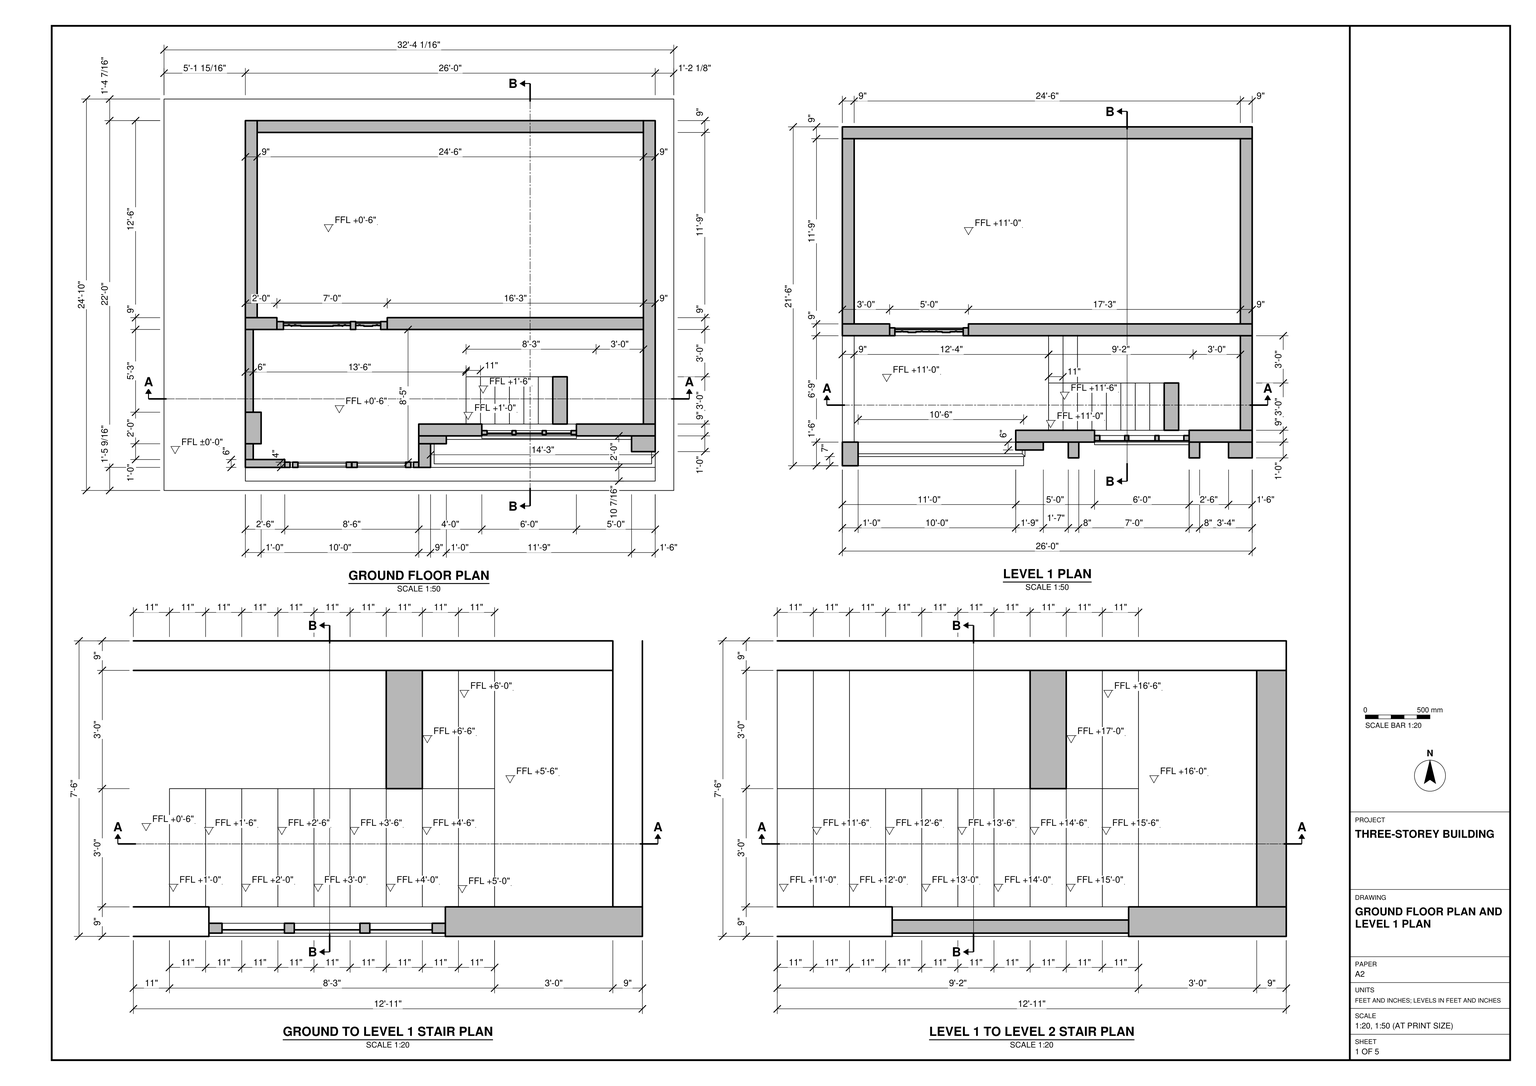
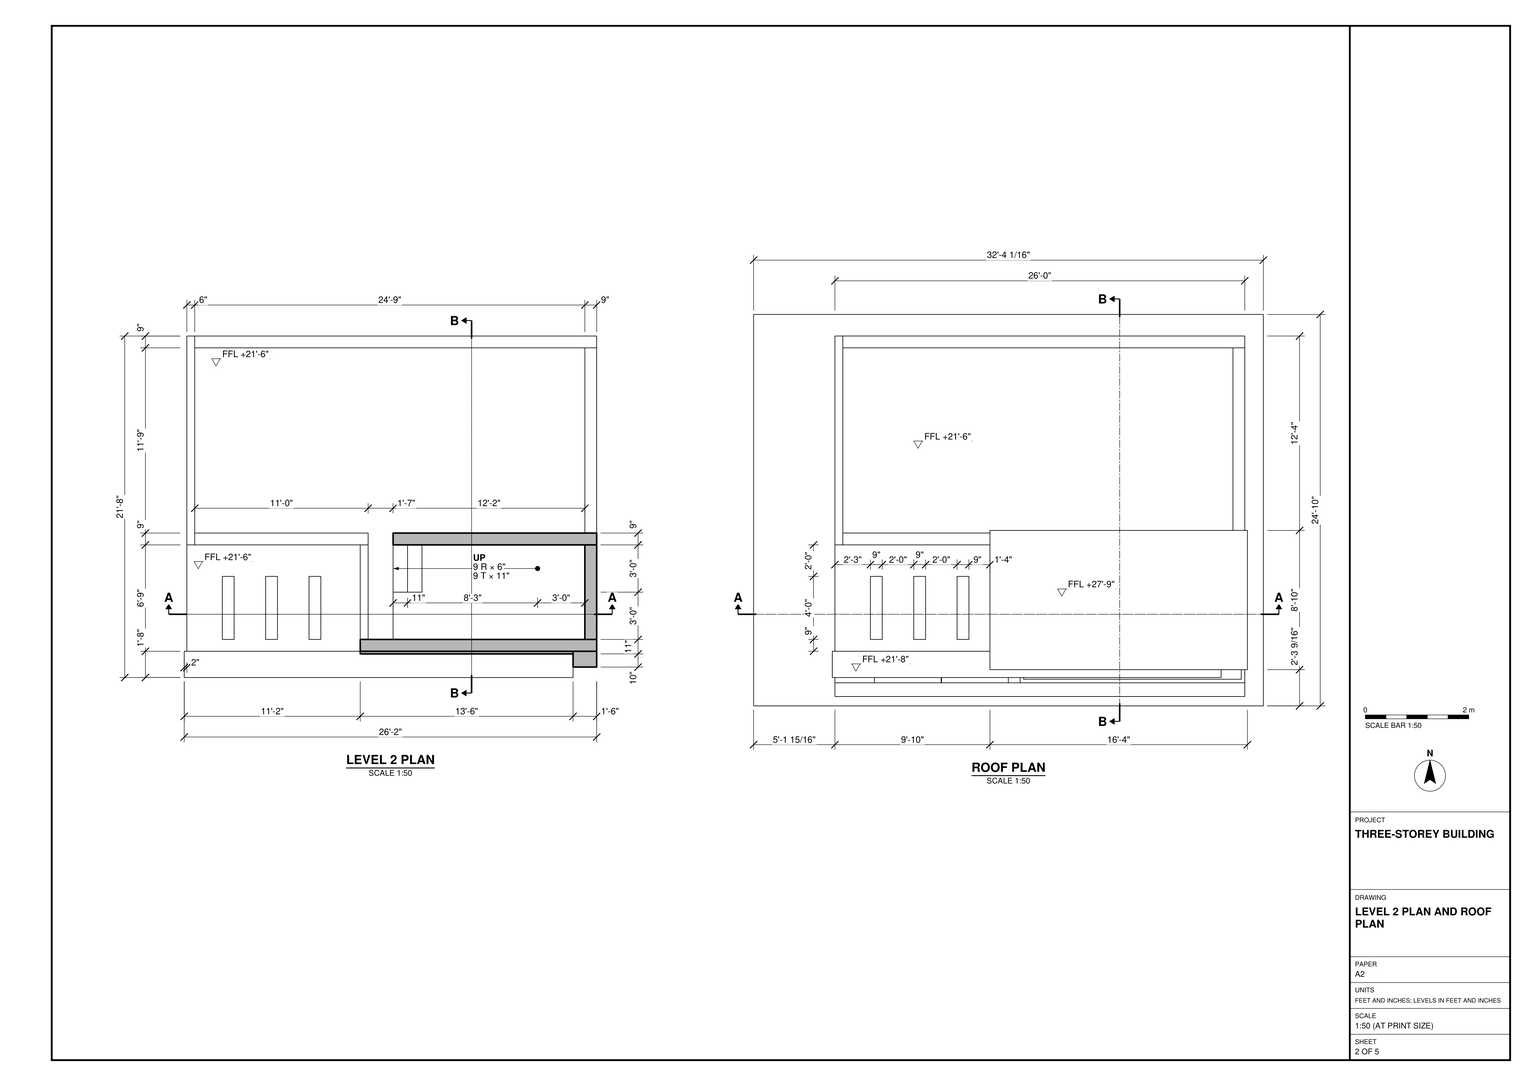
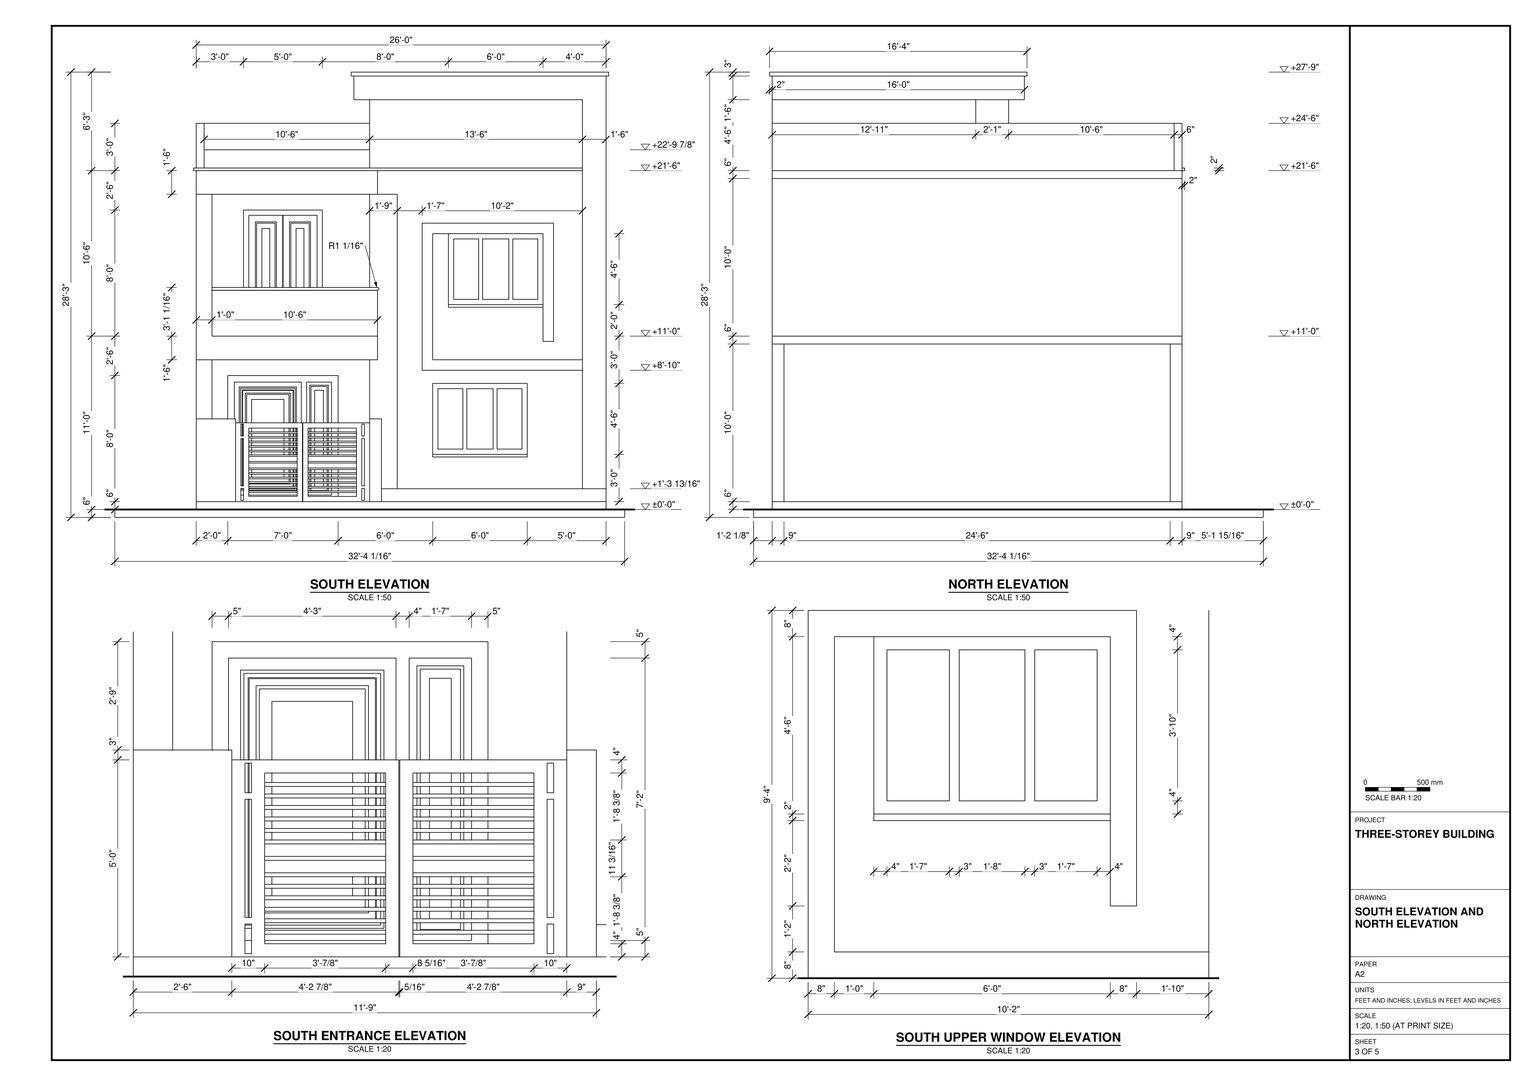
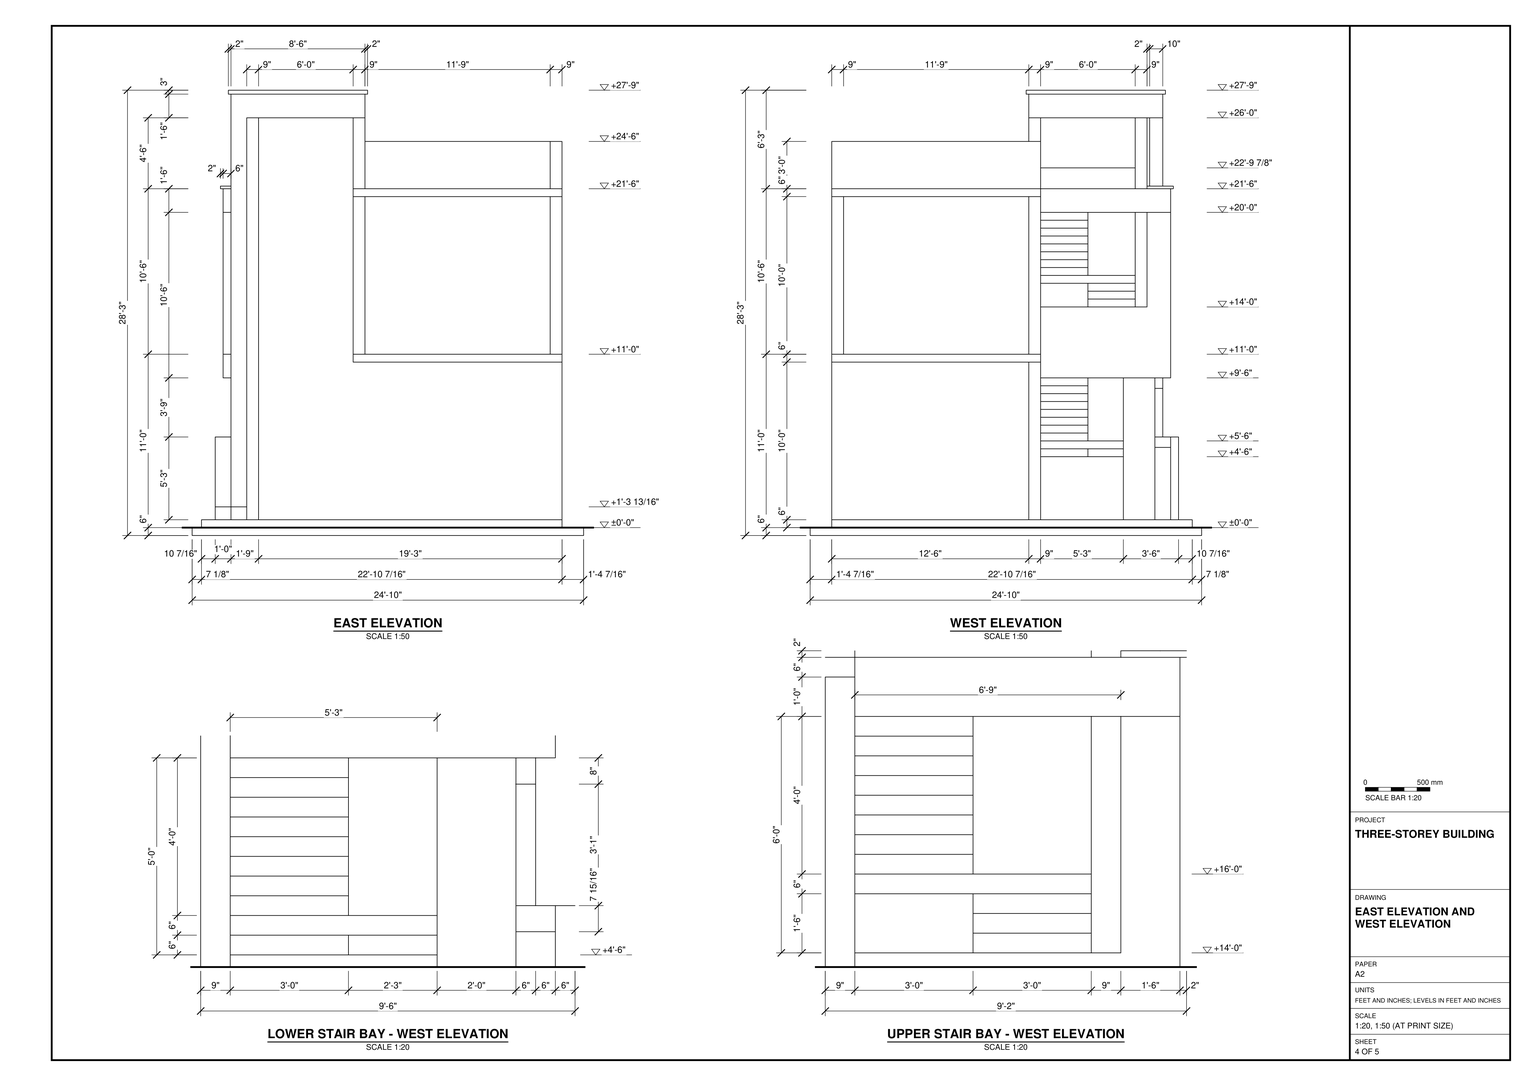
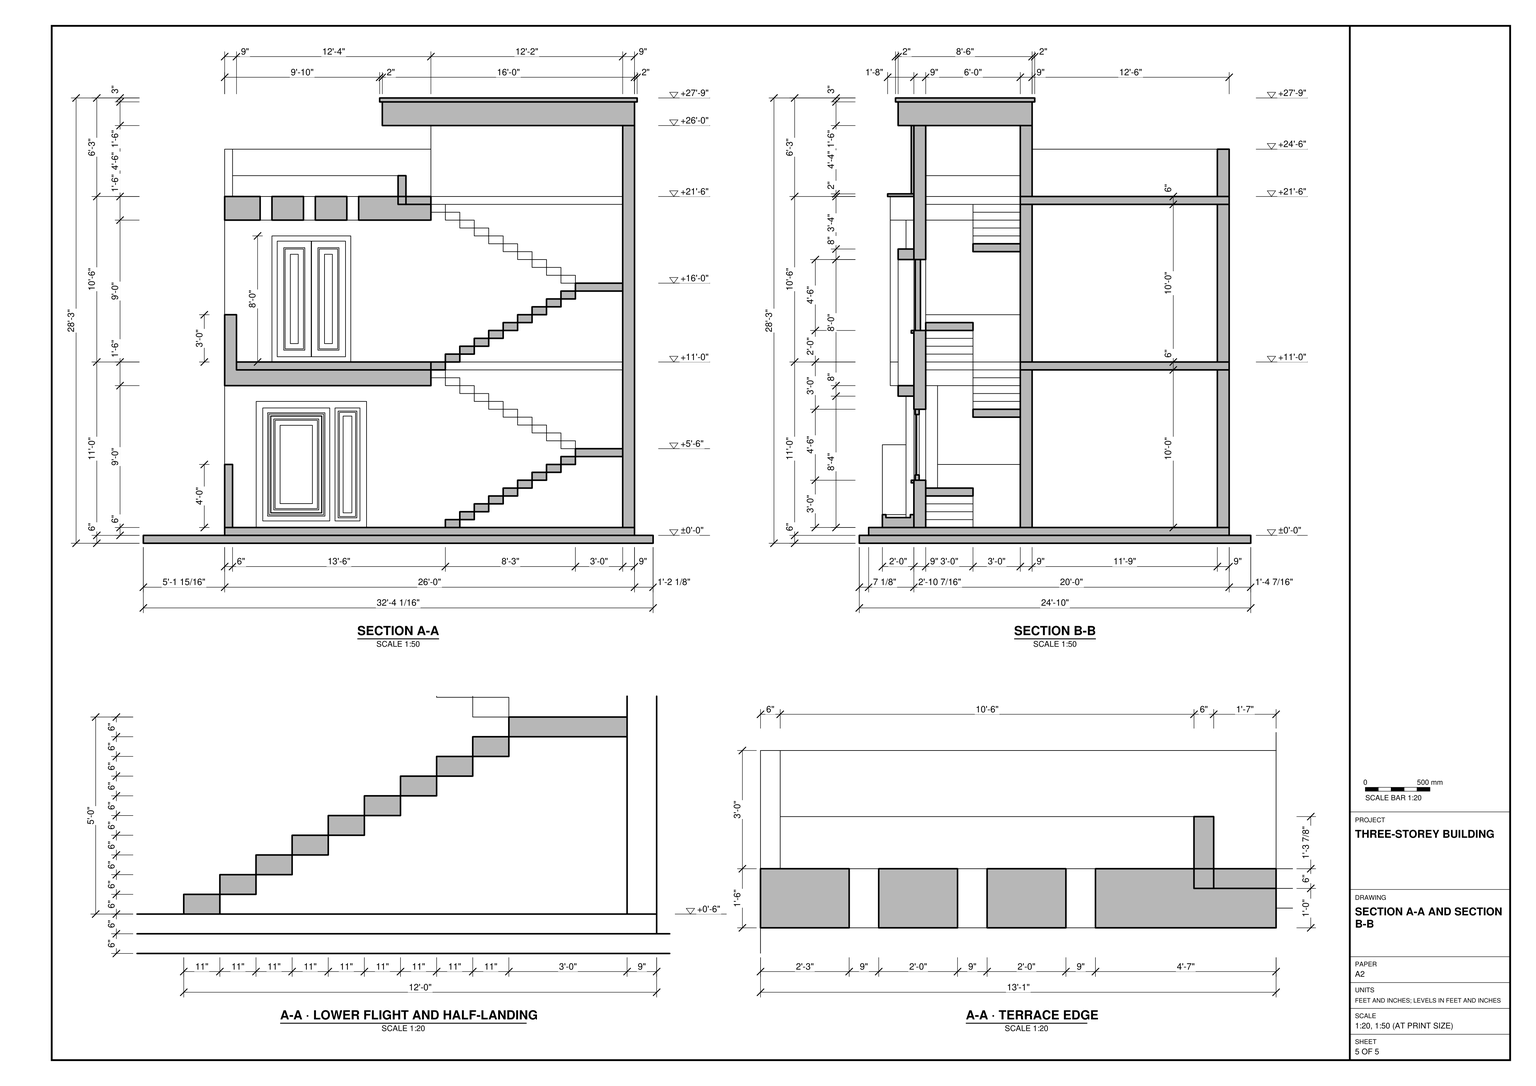
Build the three-storey building in SketchUp using task_files/diagram_01.pdf. Work in feet and inches. Including the base, the model must measure 32'-4 1/16" along X, 24'-10" along Y and 28'-3" along Z. Use ±0'-0" as the ground datum, with Level 1 at +11'-0" and Level 2 at +21'-6". Set the ground-floor finished surface at +0'-6" where marked.

Position the 26'-0" wide building on the base with the larger side setback to the west. On the ground floor and Level 1, form the full-width rear room and the front entrance and stair bays. Model the slabs and walls at their drawn thicknesses, distinguishing the 9" walls from the 6" walls. Follow the separate stair plans for the returning flights and landings so the stairs connect both floors to the roof terrace.

On the south elevation, place the slatted entrance gate in front of the recessed doorway and the balcony above it. Model the divided windows in the right-hand bay, including the projecting surround at the upper window. Finish the terrace with its parapets and the raised flat roof over the stair.

Keep walls, slabs, stairs, roof elements and any furniture or joinery pieces in separate groups or components; use components for repeated parts. Any decor or loose items shown may be suitable library components. Save one SketchUp model as output_files/three_storey_building_with_its_stair_and_roof_terrace.skp.

# SketchUp Ruby script. Lengths in inches.
U = 1.inch
M = Sketchup.active_model
def pt(a) = Geom::Point3d.new(a.map { |v| v * U })
def face(e, loops, mat)
  f = e.add_face(loops[0].map { |a| pt(a) })
  loops[1..].each { |l| e.add_face(l.map { |a| pt(a) }).erase! }
  f.material = f.back_material = mat if mat
  f
end
# faces: each face lists its corners as indices into pts; further lists are holes
def faces(e, pts, list, mat = nil) = list.each { |f| face(e, (f[0].is_a?(Array) ? f : [f]).map { |l| l.map { |i| pts[i] } }, mat) }
# xy, xz, yz: faces in a plane at the given z, y or x. An outline is a flat list of corners, or four numbers for a rectangle; further outlines are holes
def ring(l) = l.size == 4 ? [[l[0], l[1]], [l[2], l[1]], [l[2], l[3]], [l[0], l[3]]] : l.each_slice(2).to_a
def flat(e, list, mat, &to3) = list.each { |f| face(e, (f[0].is_a?(Array) ? f : [f]).map { |l| ring(l).map { |u, v| to3.(u, v) } }, mat) }
def xy(e, z, list, mat = nil) = flat(e, list, mat) { |x, y| [x, y, z] }
def xz(e, y, list, mat = nil) = flat(e, list, mat) { |x, z| [x, y, z] }
def yz(e, x, list, mat = nil) = flat(e, list, mat) { |y, z| [x, y, z] }
def lines(e, pts, list) = list.each { |a, b| e.add_line(pt(pts[a]), pt(pts[b])) }
# prism: a flat outline (further loops are holes) pulled along v
def prism(e, loops, v, mat = nil)
  f = face(e, loops, mat); d = Geom::Vector3d.new(v.map { |x| x * U })
  f.pushpull(f.normal.samedirection?(d) ? d.length : -d.length)
end
def box(e, o, s, mat = nil) = prism(e, [[o, [o[0] + s[0], o[1], o[2]], [o[0] + s[0], o[1] + s[1], o[2]], [o[0], o[1] + s[1], o[2]]]], [0, 0, s[2]], mat)
def at(x, y, z, deg = 0) = Geom::Transformation.translation(pt([x, y, z])) * Geom::Transformation.rotation(ORIGIN, Z_AXIS, deg.degrees)
def axes(o, x, y, z) = Geom::Transformation.new([*x, 0, *y, 0, *z, 0, *pt(o).to_a, 1])
def part(name) = M.definitions.add(name)
# library, detail: a bought-in or finely detailed component or shape, given as its bounding box
def library(name, o, s) = part(name).tap { |d| box(d.entities, o, s) }
def detail(e, o, s) = box(e.add_group.entities, o, s)
def put(e, d, t, mat = nil) = e.add_instance(d, t).tap { |i| i.material = mat if mat }
def group(e, t, mat = nil) = e.add_group.tap { |g| g.transformation = t; g.material = mat if mat }.entities
root = M.entities
M.materials.add("[Color E01]").color = [255, 255, 204]
M.materials.add("[Color M00]").color = [255, 255, 255]
M.materials.add("[Color M06]").color = [86, 86, 86]
M.materials.add("[Color M07]").color = [58, 58, 58]
M.materials.add("[Color M08]").color = [30, 30, 30]
M.materials.add("[Concrete Block Retaining Gray]").color = [121, 121, 121]
M.materials.add("[Grass Dark Green]").color = [106, 157, 55]
M.materials.add("[Pavers Modular Brick]").color = [158, 100, 89]
M.materials.add("[Translucent Glass Blue]").color = [100, 149, 237]
M.materials["[Translucent Glass Blue]"].alpha = 0.5
M.materials.add("[Wood Veneer 01]").color = [86, 50, 26]
c1 = part("Group\#5")
box(c1.entities,[0,0,0],[36,72,6])
c2 = part("Group\#4")
box(c2.entities,[0,0,0],[11,36,6])
c3 = part("Group\#60")
box(c3.entities,[0,1,0],[36.85,2,1.2])
c4 = part("Group\#58")
box(c4.entities,[0,1,0],[36.85,2,1.2])
c5 = part("Group\#62")
box(c5.entities,[0,1,0],[36.85,2,1.2])
c6 = part("Group\#59")
box(c6.entities,[0,1,0],[36.85,2,1.2])
p = [[199.92,35.57,138],[193.92,35.57,138],[193.92,41.57,138],[73.92,31.63,174],[199.92,31.63,174],[199.92,35.57,174],
  [199.92,35.57,120],[193.92,35.57,120],[193.92,50.57,120],[199.92,50.57,120]]
lines(root,p,[[0,1],[1,2],[3,4],[4,5],[6,7],[7,8],[8,9],[0,6]])
g1 = group(root,at(72,33,0))
box(g1,[-72,-33,0],[388.0625,298,6])
g2 = group(root,at(229.92,41.57,12),"[Color M06]")
prism(g2,[[[-36,0,0],[144,0,0],[144,0,306],[-36,0,306]],[[12,0,90],[84,0,90],[84,0,36],[12,0,36]],[[24,0,150],[24,0,204],[96,0,204],[96,0,150]]],[0,9,0])
g3 = group(root,at(364.92,50.57,12),"[Color E01]")
prism(g3,[[[0,231,0],[0,0,0],[0,0,306],[0,72,306],[0,72,120],[0,231,120]]],[9,0,0])
g4 = group(root,at(109.92,122.57,12),"[Color E01]")
prism(g4,[[[255,9,120],[255,9,0],[60,9,0],[60,9,96],[-24,9,96],[-24,9,0],[-48,9,0],[-48,9,120]]],[0,-9,0])
g5 = group(root,at(218.92,50.57,12))
put(g5,c1,at(110,0,54))
g6 = group(g5,at(11,0,0))
put(g6,c2,at(66,0,36))
put(g6,c2,at(88,0,48))
put(g6,c2,at(0,0,0))
put(g6,c2,at(77,0,42))
put(g6,c2,at(11,0,6))
put(g6,c2,at(55,0,30))
put(g6,c2,at(22,0,12))
put(g6,c2,at(33,0,18))
put(g6,c2,at(44,0,24))
put(g5,c2,at(22,72,108,180))
put(g5,c2,at(55,72,90,180))
put(g5,c2,at(44,72,96,180))
put(g5,c2,at(99,72,66,180))
put(g5,c2,at(110,72,60,180))
put(g5,c2,at(77,72,78,180))
put(g5,c2,at(33,72,102,180))
put(g5,c2,at(88,72,72,180))
put(g5,c2,at(66,72,84,180))
put(g5,c2,at(11,72,114,180))
g7 = group(root,at(109.92,122.57,132),"[Color E01]")
prism(g7,[[[264,0,0],[109,0,0],[109,-72,0],[84,-72,0],[84,-81,0],[-39,-81,0],[-39,0,0],[-48,0,0],[-48,159,0],[264,159,0]]],[0,0,6])
put(root,c2,at(317.92,122.57,204,180))
put(root,c2,at(273.92,122.57,228,180))
put(root,c2,at(251.92,122.57,240,180))
put(root,c2,at(240.92,122.57,246,180))
put(root,c2,at(284.92,122.57,222,180))
put(root,c2,at(306.92,122.57,210,180))
put(root,c2,at(295.92,122.57,216,180))
put(root,c2,at(328.92,122.57,198,180))
put(root,c2,at(262.92,122.57,234,180))
put(root,c1,at(328.92,50.57,192))
put(root,c2,at(229.92,122.57,252,180))
put(root,c2,at(295.92,50.57,174))
put(root,c2,at(240.92,50.57,144))
put(root,c2,at(251.92,50.57,150))
put(root,c2,at(262.92,50.57,156))
put(root,c2,at(317.92,50.57,186))
put(root,c2,at(284.92,50.57,168))
put(root,c2,at(273.92,50.57,162))
put(root,c2,at(229.92,50.57,138))
put(root,c2,at(306.92,50.57,180))
put(root,c2,at(218.92,50.57,132))
g8 = group(root,at(109.92,122.57,138),"[Color E01]")
prism(g8,[[[-12,9,0],[-48,9,0],[-48,9,120],[264,9,120],[264,9,0],[48,9,0],[48,9,96],[-12,9,96]]],[0,-9,0])
g9 = group(root,at(109.92,272.57,138),"[Color E01]")
box(g9,[-48,0,0],[312,9,120])
g10 = group(root,at(364.92,131.57,138),"[Color E01]")
box(g10,[0,0,0],[9,141,120])
g11 = group(root,at(109.92,122.57,258),"[Color E01]")
prism(g11,[[[264,159,0],[264,0,0],[109,0,0],[109,-72,0],[84,-72,0],[84,0,0],[-48,0,0],[-48,159,0]]],[0,0,6])
g12 = group(root,at(241.92,41.57,48),"[Color M08]")
prism(g12,[[[0,4,54],[72,4,54],[72,4,0],[0,4,0]],[[26,4,4],[46,4,4],[46,4,50],[26,4,50]],[[23,4,4],[23,4,50],[4,4,50],[4,4,4]],[[49,4,50],[49,4,4],[68,4,4],[68,4,50]]],[0,-3,0])
g13 = group(root,at(290.92,43.57,52),"[Translucent Glass Blue]")
xz(g13,0,[[0,0,19,46]])
g14 = group(root,at(267.92,43.57,52),"[Translucent Glass Blue]")
xz(g14,0,[[0,0,20,46]])
g15 = group(root,at(245.92,43.57,52),"[Translucent Glass Blue]")
xz(g15,0,[[0,0,19,46]])
g16 = group(root,at(109.92,41.57,120),"[Color E01]")
xy(g16,0,[[-48,-18,-48,81,109,81,109,9,90,9,90,-18]])
xy(g16,12,[[-39,0,90,0,90,9,109,9,109,81,-39,81]])
xy(g16,18,[[-36,-18,90,0]])
xy(g16,54,[[-48,0,-39,81]])
xy(g16,126,[[-48,-18,-36,0]])
xz(g16,-18,[[-48,0,90,0,90,18,-36,18,-36,126,-48,126]])
xz(g16,0,[[-39,12,-39,54,-48,54,-48,126,-36,126,-36,18,90,18,90,12]])
xz(g16,9,[[90,0,109,12]])
xz(g16,81,[[-48,0,-48,54,-39,54,-39,12,109,12,109,0]])
yz(g16,-48,[[-18,0,-18,126,0,126,0,54,81,54,81,0]])
yz(g16,-39,[[0,12,81,54]])
yz(g16,-36,[[-18,18,0,126]])
yz(g16,90,[[-18,0,9,0,9,12,0,12,0,18,-18,18]])
yz(g16,109,[[9,0,81,12]])
g17 = group(root,at(85.92,122.57,12),"[Wood Veneer 01]")
prism(g17,[[[84,6,0],[0,6,0],[0,6,96],[84,6,96]],[[56,6,5],[56,6,91],[5,6,91],[5,6,5]],[[79,6,91],[60,6,91],[60,6,5],[79,6,5]]],[0,-6,0])
g18 = group(root,at(90.92,125.07,17),"[Wood Veneer 01]")
xy(g18,0,[[0,0.5,51,2.5]])
xy(g18,3.67,[[3.67,0.5,47.33,1]])
xy(g18,4.67,[[4.67,0.5,46.33,1]])
xy(g18,5.96,[[5.96,0,45.04,0.5]])
xy(g18,6.28,[[6.28,0,44.72,0.5]])
xy(g18,8.39,[[8.39,0.5,42.61,1]])
xy(g18,9.39,[[9.39,0.5,41.61,1]])
xy(g18,13.2,[[13.2,0,37.8,0.5]])
xy(g18,72.8,[[13.2,0,37.8,0.5]])
xy(g18,76.61,[[9.39,0.5,41.61,1]])
xy(g18,77.61,[[8.39,0.5,42.61,1]])
xy(g18,79.72,[[6.28,0,44.72,0.5]])
xy(g18,80.04,[[5.96,0,45.04,0.5]])
xy(g18,81.33,[[4.67,0.5,46.33,1]])
xy(g18,82.33,[[3.67,0.5,47.33,1]])
xy(g18,86,[[0,0.5,51,2.5]])
xz(g18,0,[[[5.96,5.96,45.04,80.04],[6.28,6.28,44.72,79.72]],[13.2,13.2,37.8,72.8]])
xz(g18,0.5,[[[0,0,51,86],[3.67,3.67,47.33,82.33]],[[4.67,4.67,46.33,81.33],[5.96,5.96,45.04,80.04]],[[6.28,6.28,44.72,79.72],[8.39,8.39,42.61,77.61]],[[9.39,9.39,41.61,76.61],[13.2,13.2,37.8,72.8]]])
xz(g18,1,[[[3.67,3.67,47.33,82.33],[4.67,4.67,46.33,81.33]],[[8.39,8.39,42.61,77.61],[9.39,9.39,41.61,76.61]]])
xz(g18,2.5,[[0,0,51,86]])
yz(g18,0,[[0.5,0,2.5,86]])
yz(g18,3.67,[[0.5,3.67,1,82.33]])
yz(g18,4.67,[[0.5,4.67,1,81.33]])
yz(g18,5.96,[[0,5.96,0.5,80.04]])
yz(g18,6.28,[[0,6.28,0.5,79.72]])
yz(g18,8.39,[[0.5,8.39,1,77.61]])
yz(g18,9.39,[[0.5,9.39,1,76.61]])
yz(g18,13.2,[[0,13.2,0.5,72.8]])
yz(g18,37.8,[[0,13.2,0.5,72.8]])
yz(g18,41.61,[[0.5,9.39,1,76.61]])
yz(g18,42.61,[[0.5,8.39,1,77.61]])
yz(g18,44.72,[[0,6.28,0.5,79.72]])
yz(g18,45.04,[[0,5.96,0.5,80.04]])
yz(g18,46.33,[[0.5,4.67,1,81.33]])
yz(g18,47.33,[[0.5,3.67,1,82.33]])
yz(g18,51,[[0.5,0,2.5,86]])
g19 = group(root,at(145.92,125.07,17),"[Wood Veneer 01]")
xy(g19,0,[[0,0.5,19,2.5]])
xy(g19,2.37,[[2.37,0.5,16.63,1]])
xy(g19,3.37,[[3.37,0.5,15.63,1]])
xy(g19,6.17,[[6.17,0,12.83,0.5]])
xy(g19,79.83,[[6.17,0,12.83,0.5]])
xy(g19,82.63,[[3.37,0.5,15.63,1]])
xy(g19,83.63,[[2.37,0.5,16.63,1]])
xy(g19,86,[[0,0.5,19,2.5]])
xz(g19,0,[[6.17,6.17,12.83,79.83]])
xz(g19,0.5,[[[0,0,19,86],[2.37,2.37,16.63,83.63]],[[3.37,3.37,15.63,82.63],[6.17,6.17,12.83,79.83]]])
xz(g19,1,[[[2.37,2.37,16.63,83.63],[3.37,3.37,15.63,82.63]]])
xz(g19,2.5,[[0,0,19,86]])
yz(g19,0,[[0.5,0,2.5,86]])
yz(g19,2.37,[[0.5,2.37,1,83.63]])
yz(g19,3.37,[[0.5,3.37,1,82.63]])
yz(g19,6.17,[[0,6.17,0.5,79.83]])
yz(g19,12.83,[[0,6.17,0.5,79.83]])
yz(g19,15.63,[[0.5,3.37,1,82.63]])
yz(g19,16.63,[[0.5,2.37,1,83.63]])
yz(g19,19,[[0.5,0,2.5,86]])
g20 = group(root,at(355.92,29.57,12))
xy(g20,0,[[0,0,18,12]])
xy(g20,306,[[-174,0,0,102],[0,12,18,102]])
xy(g20,324,[[-174,0,18,102]])
xz(g20,0,[[0,0,18,0,18,324,-174,324,-174,306,0,306]])
xz(g20,12,[[0,0,18,306]])
xz(g20,102,[[-174,306,18,324]])
yz(g20,-174,[[0,306,102,324]])
yz(g20,0,[[0,0,12,306]])
yz(g20,18,[[0,0,12,0,12,306,102,306,102,324,0,324]])
g21 = group(root,at(233.92,29.57,112))
prism(g21,[[[122,0,8],[8,0,8],[8,0,104],[92,0,104],[92,0,22],[100,0,22],[100,0,112],[0,0,112],[0,0,0],[122,0,0]]],[0,12,0])
g22 = group(root,at(253.92,42.57,162),"[Color M08]")
prism(g22,[[[0,0,54],[0,0,0],[72,0,0],[72,0,54]],[[26,0,4],[26,0,50],[46,0,50],[46,0,4]],[[49,0,4],[49,0,50],[68,0,50],[68,0,4]],[[23,0,4],[4,0,4],[4,0,50],[23,0,50]]],[0,4,0])
g23 = group(root,at(302.92,42.57,166),"[Translucent Glass Blue]")
xz(g23,0,[[0,0,19,46]])
g24 = group(root,at(279.92,42.57,166),"[Translucent Glass Blue]")
xz(g24,0,[[0,0,20,46]])
g25 = group(root,at(257.92,42.57,166),"[Translucent Glass Blue]")
xz(g25,0,[[0,0,19,46]])
g26 = group(root,at(61.92,50.57,246),"[Color E01]")
xy(g26,0,[[[0,-27,0,72,157,72,157,0,138,0,138,-27],[27,0,36,48],[93,0,102,48],[60,0,69,48]]])
xy(g26,12,[[138,0,157,72]])
xy(g26,18,[[[0,-27,138,72],[27,0,36,48],[93,0,102,48],[60,0,69,48]]])
xz(g26,-27,[[0,0,138,18]])
xz(g26,0,[[27,0,36,18],[60,0,69,18],[93,0,102,18],[138,0,157,12]])
xz(g26,48,[[27,0,36,18],[60,0,69,18],[93,0,102,18]])
xz(g26,72,[[0,0,157,12],[0,12,138,18]])
yz(g26,0,[[-27,0,72,18]])
yz(g26,27,[[0,0,48,18]])
yz(g26,36,[[0,0,48,18]])
yz(g26,60,[[0,0,48,18]])
yz(g26,69,[[0,0,48,18]])
yz(g26,93,[[0,0,48,18]])
yz(g26,102,[[0,0,48,18]])
yz(g26,138,[[-27,0,0,0,0,12,72,12,72,18,-27,18]])
yz(g26,157,[[0,0,72,12]])
g27 = group(root,at(97.92,122.57,138),"[Wood Veneer 01]")
prism(g27,[[[0,6,0],[0,6,96],[60,6,96],[60,6,0]],[[56,6,92],[4,6,92],[4,6,4],[56,6,4]]],[0,-6,0])
g28 = group(root,at(101.92,125.57,142),"[Wood Veneer 01]")
xy(g28,0,[[0,0,0,2,52,2,52,0,26.15,0,26.15,0.5,25.85,0.5,25.85,0]])
xy(g28,5,[[5,0,21,0.5],[31,0,47,0.5]])
xy(g28,6,[[6,0,20,0.5],[32,0,46,0.5]])
xy(g28,10,[[10,-0.5,16,0],[36,-0.5,42,0]])
xy(g28,78,[[10,-0.5,16,0],[36,-0.5,42,0]])
xy(g28,82,[[6,0,20,0.5],[32,0,46,0.5]])
xy(g28,83,[[5,0,21,0.5],[31,0,47,0.5]])
xy(g28,88,[[0,0,25.85,0,25.85,0.5,26.15,0.5,26.15,0,52,0,52,2,0,2]])
xz(g28,-0.5,[[10,10,16,78],[36,10,42,78]])
xz(g28,0,[[[0,0,25.85,88],[5,5,21,83]],[[26.15,0,52,88],[31,5,47,83]],[[6,6,20,82],[10,10,16,78]],[[32,6,46,82],[36,10,42,78]]])
xz(g28,0.5,[[25.85,0,26.15,88],[[5,5,21,83],[6,6,20,82]],[[31,5,47,83],[32,6,46,82]]])
xz(g28,2,[[0,0,52,88]])
yz(g28,0,[[0,0,2,88]])
yz(g28,5,[[0,5,0.5,83]])
yz(g28,6,[[0,6,0.5,82]])
yz(g28,10,[[-0.5,10,0,78]])
yz(g28,16,[[-0.5,10,0,78]])
yz(g28,20,[[0,6,0.5,82]])
yz(g28,21,[[0,5,0.5,83]])
yz(g28,25.85,[[0,0,0.5,88]])
yz(g28,26.15,[[0,0,0.5,88]])
yz(g28,31,[[0,5,0.5,83]])
yz(g28,32,[[0,6,0.5,82]])
yz(g28,36,[[-0.5,10,0,78]])
yz(g28,42,[[-0.5,10,0,78]])
yz(g28,46,[[0,6,0.5,82]])
yz(g28,47,[[0,5,0.5,83]])
yz(g28,52,[[0,0,2,88]])
g29 = group(root,at(253.92,39.57,160))
box(g29,[0,0,0],[72,2,2])
g30 = group(root,at(241.92,39.57,46))
box(g30,[0,0,0],[72,2,2])
g31 = group(root,at(218.92,122.57,264),"[Color E01]")
box(g31,[0,0,0],[155,9,54])
g32 = group(root,at(193.92,35.57,12),"[Pavers Modular Brick]")
box(g32,[0,0,0],[21,6,234],"[Pavers Modular Brick]")
g33 = group(root,at(73.92,30.57,172.9375),"[Color M07]")
xz(g33,5,[[125.94,0,125.67,0.05,125.42,0.17,125.21,0.35,125.05,0.58,124.96,0.84,124.9375,1.12,124.99,1.39,125.11,1.64,125.29,1.85,125.52,2.01,125.78,2.1,126.06,2.12,126.33,2.07,126.58,1.95,126.79,1.77,126.95,1.54,127.04,1.28,127.0625,1.01,127.01,0.73,126.89,0.48,126.71,0.27,126.48,0.11,126.22,0.02]])
yz(g33,0,[[1.12,0,0.84,0.02,0.58,0.11,0.35,0.27,0.17,0.48,0.05,0.73,0,1.01,0.02,1.28,0.11,1.54,0.27,1.77,0.48,1.95,0.73,2.07,1.01,2.12,1.28,2.1,1.54,2.01,1.77,1.85,1.95,1.64,2.07,1.39,2.12,1.12,2.1,0.84,2.01,0.58,1.85,0.35,1.64,0.17,1.39,0.05]])
p = [[0,0.58,0.11],[0,0.84,0.02],[126.22,0.84,0.02],[126.48,0.58,0.11],[126.22,5,0.02],[126.48,5,0.11],
  [0,1.12,0],[125.94,1.12,0],[125.94,5,0],[0,1.39,0.05],[125.67,1.39,0.05],[125.67,5,0.05],
  [0,0.35,0.27],[126.71,0.35,0.27],[126.71,5,0.27],[0,1.64,0.17],[125.42,1.64,0.17],[125.42,5,0.17],
  [0,1.85,0.35],[125.21,1.85,0.35],[125.21,5,0.35],[0,0.17,0.48],[126.89,0.17,0.48],[126.89,5,0.48],
  [0,2.01,0.58],[125.05,2.01,0.58],[125.05,5,0.58],[0,0.05,0.73],[127.01,0.05,0.73],[127.01,5,0.73],
  [0,2.1,0.84],[124.96,2.1,0.84],[124.96,5,0.84],[0,0,1.01],[127.0625,0,1.01],[127.0625,5,1.01],
  [0,2.12,1.12],[124.9375,2.12,1.12],[124.9375,5,1.12],[0,0.02,1.28],[127.04,0.02,1.28],[127.04,5,1.28],
  [0,2.07,1.39],[124.99,2.07,1.39],[124.99,5,1.39],[0,0.11,1.54],[126.95,0.11,1.54],[126.95,5,1.54],
  [0,1.95,1.64],[125.11,1.95,1.64],[125.11,5,1.64],[0,0.27,1.77],[126.79,0.27,1.77],[126.79,5,1.77],
  [0,1.77,1.85],[125.29,1.77,1.85],[125.29,5,1.85],[0,0.48,1.95],[126.58,0.48,1.95],[126.58,5,1.95],
  [0,1.54,2.01],[125.52,1.54,2.01],[125.52,5,2.01],[0,0.73,2.07],[126.33,0.73,2.07],[126.33,5,2.07],
  [0,1.28,2.1],[125.78,1.28,2.1],[125.78,5,2.1],[0,1.01,2.12],[126.06,1.01,2.12],[126.06,5,2.12]]
faces(g33,p,[[0,1,2,3],[3,2,4,5],[1,6,7,2],[2,7,8,4],[6,9,10,7],[7,10,11,8],[12,0,3,13],[13,3,5,14],
  [9,15,16,10],[10,16,17,11],[15,18,19,16],[16,19,20,17],[21,12,13,22],[22,13,14,23],[18,24,25,19],[19,25,26,20],
  [27,21,22,28],[28,22,23,29],[24,30,31,25],[25,31,32,26],[33,27,28,34],[34,28,29,35],[30,36,37,31],[31,37,38,32],
  [39,33,34,40],[40,34,35,41],[36,42,43,37],[37,43,44,38],[45,39,40,46],[46,40,41,47],[42,48,49,43],[43,49,50,44],
  [51,45,46,52],[52,46,47,53],[48,54,55,49],[49,55,56,50],[57,51,52,58],[58,52,53,59],[54,60,61,55],[55,61,62,56],
  [63,57,58,64],[64,58,59,65],[60,66,67,61],[61,67,68,62],[69,63,64,70],[70,64,65,71],[66,69,70,67],[67,70,71,68]])
g34 = group(root,at(73.92,31.63,138),"[Translucent Glass Blue]")
xz(g34,0,[[0,0,126,34.85]])
g35 = group(root,at(199.92,31.63,138.22),"[Translucent Glass Blue]")
yz(g35,0,[[0,0,3.75,34.625]])
g36 = group(root,at(61.92,23.57,264))
box(g36,[-2,-2,0],[296,20,2])
g37 = group(root,at(193.92,39.57,266),"[Concrete Block Retaining Gray]")
box(g37,[0,0,0],[162,2,52])
g38 = group(root,at(61.92,35.57,12),"[Color E01]")
box(g38,[0,0,0],[12,24,108])
g39 = group(root,at(61.92,131.57,12),"[Color E01]")
box(g39,[0,0,0],[9,150,120])
g40 = group(root,at(70.92,272.57,12),"[Color E01]")
box(g40,[0,0,0],[294,9,120])
g41 = group(root,at(61.92,131.57,138),"[Color E01]")
box(g41,[0,0,0],[9,141,120])
g42 = group(root,at(181.92,29.57,336),"[Color M08]")
box(g42,[-2,-2,0],[196,106,3])
g43 = group(root,at(61.92,59.57,12),"[Color E01]")
box(g43,[0,0,0],[6,63,48])
g44 = group(root,at(193.92,17.57,12),"[Color E01]")
box(g44,[0,0,0],[9,18,63])
g45 = group(root,at(61.92,17.57,12),"[Color E01]")
box(g45,[0,0,0],[30,6,63])
g46 = group(root,at(61.92,23.57,12),"[Color E01]")
box(g46,[0,0,0],[6,12,55.0625])
g47 = group(root,at(61.92,122.57,264),"[Color E01]")
box(g47,[0,0,0],[6,159,36])
g48 = group(root,at(67.92,272.57,264),"[Color E01]")
box(g48,[0,0,0],[306,9,36])
g49 = group(root,at(364.92,131.57,264),"[Color E01]")
box(g49,[0,0,0],[9,141,36])
g50 = group(root,at(193.92,50.57,264),"[Color E01]")
box(g50,[0,0,0],[6,72,15.875])
g51 = group(root,at(67.92,122.57,264),"[Color E01]")
box(g51,[0,0,0],[132,9,15.875])
g52 = group(root,at(202.92,17.57,12),"[Color M00]")
xy(g52,0,[[0,0,171,24]])
xy(g52,7.5625,[[2.71,2.71,168.29,21.29]],"[Grass Dark Green]")
xy(g52,9.8125,[[[0,0,171,24],[2.71,2.71,168.29,21.29]]])
xz(g52,0,[[0,0,171,9.8125]])
xz(g52,2.71,[[2.71,7.5625,168.29,9.8125]])
xz(g52,21.29,[[2.71,7.5625,168.29,9.8125]])
xz(g52,24,[[0,0,171,9.8125]])
yz(g52,0,[[0,0,24,9.8125]])
yz(g52,2.71,[[2.71,7.5625,21.29,9.8125]])
yz(g52,168.29,[[2.71,7.5625,21.29,9.8125]])
yz(g52,171,[[0,0,24,9.8125]])
g53 = group(root,at(109.92,41.57,6))
box(g53,[-48,-34.4375,0],[312,274.4375,6])
g54 = group(root,at(91.92,17.57,12),"[Color M08]")
xy(g54,0,[[0,0,10,4],[10,0,50.85,4]])
xy(g54,1,[[4,0,6,4]])
xy(g54,4,[[10,0,46.85,4]])
xy(g54,10,[[4,0,6,4]])
xy(g54,12,[[4,0,6,4]])
xy(g54,48,[[4,0,6,4]])
xy(g54,50,[[4,0,6,4]])
xy(g54,56,[[10,0,46.85,4]])
xy(g54,59,[[4,0,6,4]])
xy(g54,60,[[0,0,50.85,4]])
xz(g54,0,[[[0,0,50.85,60],[10,4,46.85,56],[4,12,6,48],[4,1,6,10],[4,50,6,59]]])
xz(g54,4,[[[0,0,0,60,50.85,60,50.85,0,10,0,10,4,46.85,4,46.85,56,10,56,10,0],[4,12,6,48],[4,1,6,10],[4,50,6,59]]])
yz(g54,0,[[0,0,4,60]])
yz(g54,4,[[0,1,4,10],[0,12,4,48],[0,50,4,59]])
yz(g54,6,[[0,1,4,10],[0,12,4,48],[0,50,4,59]])
yz(g54,10,[[3,0,4,4],[0,4,4,56]])
yz(g54,46.85,[[0,4,4,56]])
yz(g54,50.85,[[0,0,4,60]])
g55 = group(root,at(143.07,17.57,12),"[Color M08]")
prism(g55,[[[50.85,4,0],[0,4,0],[0,4,60],[50.85,4,60]],[[40.85,4,56],[4,4,56],[4,4,4],[40.85,4,4]],[[46.85,4,12],[46.85,4,48],[44.85,4,48],[44.85,4,12]],[[46.85,4,59],[44.85,4,59],[44.85,4,50],[46.85,4,50]],[[44.85,4,1],[46.85,4,1],[46.85,4,10],[44.85,4,10]]],[0,-4,0])
g56 = group(root,at(101.92,17.57,41.4),"[Color M08]")
box(g56,[0,0,0],[36.85,3,1.2])
g57 = group(root,at(147.07,17.57,41.4),"[Color M08]")
box(g57,[0,0,0],[36.85,3,1.2])
put(root,c3,at(101.92,17.57,46.4),"[Color M08]")
put(root,c4,at(101.92,17.57,36.4),"[Color M08]")
put(root,c4,at(101.92,17.57,32.9),"[Color M08]")
put(root,c4,at(101.92,17.57,29.4),"[Color M08]")
put(root,c4,at(101.92,17.57,25.9),"[Color M08]")
put(root,c4,at(101.92,17.57,22.4),"[Color M08]")
put(root,c4,at(101.92,17.57,18.9),"[Color M08]")
put(root,c3,at(101.92,17.57,49.9),"[Color M08]")
put(root,c3,at(101.92,17.57,53.4),"[Color M08]")
put(root,c3,at(101.92,17.57,56.9),"[Color M08]")
put(root,c3,at(101.92,17.57,60.4),"[Color M08]")
put(root,c3,at(101.92,17.57,63.9),"[Color M08]")
put(root,c5,at(147.07,17.57,46.4),"[Color M08]")
put(root,c6,at(147.07,17.57,36.4),"[Color M08]")
put(root,c6,at(147.07,17.57,32.9),"[Color M08]")
put(root,c6,at(147.07,17.57,29.4),"[Color M08]")
put(root,c6,at(147.07,17.57,25.9),"[Color M08]")
put(root,c6,at(147.07,17.57,22.4),"[Color M08]")
put(root,c6,at(147.07,17.57,18.9),"[Color M08]")
put(root,c5,at(147.07,17.57,49.9),"[Color M08]")
put(root,c5,at(147.07,17.57,53.4),"[Color M08]")
put(root,c5,at(147.07,17.57,56.9),"[Color M08]")
put(root,c5,at(147.07,17.57,60.4),"[Color M08]")
put(root,c5,at(147.07,17.57,63.9),"[Color M08]")
g58 = group(root,at(147.07,20.57,36.4),"[Color M07]")
box(g58,[0,0,0],[36.85,1,11.2])
g59 = group(root,at(101.92,20.57,36.4),"[Color M07]")
box(g59,[0,0,0],[36.85,1,11.2])
